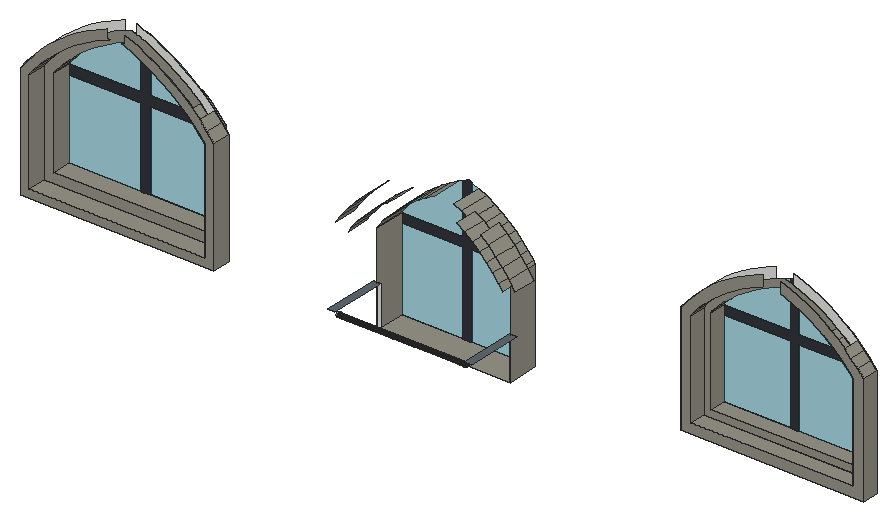
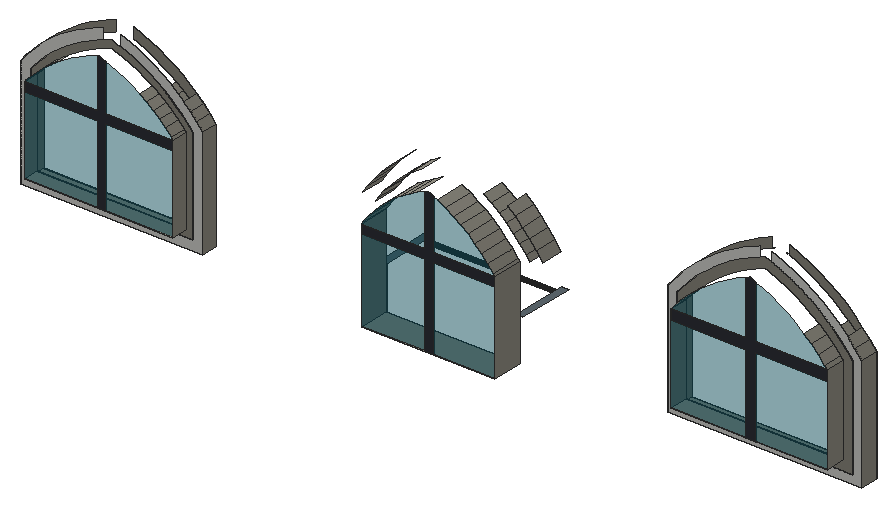
# SketchUp Ruby script. Lengths in inches.
U = 1.inch
M = Sketchup.active_model
def pt(a) = Geom::Point3d.new(a.map { |v| v * U })
def face(e, loops, mat)
  f = e.add_face(loops[0].map { |a| pt(a) })
  loops[1..].each { |l| e.add_face(l.map { |a| pt(a) }).erase! }
  f.material = f.back_material = mat if mat
  f
end
# faces: each face lists its corners as indices into pts; further lists are holes
def faces(e, pts, list, mat = nil) = list.each { |f| face(e, (f[0].is_a?(Array) ? f : [f]).map { |l| l.map { |i| pts[i] } }, mat) }
# xy, xz, yz: faces in a plane at the given z, y or x. An outline is a flat list of corners, or four numbers for a rectangle; further outlines are holes
def ring(l) = l.size == 4 ? [[l[0], l[1]], [l[2], l[1]], [l[2], l[3]], [l[0], l[3]]] : l.each_slice(2).to_a
def flat(e, list, mat, &to3) = list.each { |f| face(e, (f[0].is_a?(Array) ? f : [f]).map { |l| ring(l).map { |u, v| to3.(u, v) } }, mat) }
def xy(e, z, list, mat = nil) = flat(e, list, mat) { |x, y| [x, y, z] }
def xz(e, y, list, mat = nil) = flat(e, list, mat) { |x, z| [x, y, z] }
def yz(e, x, list, mat = nil) = flat(e, list, mat) { |y, z| [x, y, z] }
def lines(e, pts, list) = list.each { |a, b| e.add_line(pt(pts[a]), pt(pts[b])) }
# prism: a flat outline (further loops are holes) pulled along v
def prism(e, loops, v, mat = nil)
  f = face(e, loops, mat); d = Geom::Vector3d.new(v.map { |x| x * U })
  f.pushpull(f.normal.samedirection?(d) ? d.length : -d.length)
end
def box(e, o, s, mat = nil) = prism(e, [[o, [o[0] + s[0], o[1], o[2]], [o[0] + s[0], o[1] + s[1], o[2]], [o[0], o[1] + s[1], o[2]]]], [0, 0, s[2]], mat)
def at(x, y, z, deg = 0) = Geom::Transformation.translation(pt([x, y, z])) * Geom::Transformation.rotation(ORIGIN, Z_AXIS, deg.degrees)
def axes(o, x, y, z) = Geom::Transformation.new([*x, 0, *y, 0, *z, 0, *pt(o).to_a, 1])
def part(name) = M.definitions.add(name)
# library, detail: a bought-in or finely detailed component or shape, given as its bounding box
def library(name, o, s) = part(name).tap { |d| box(d.entities, o, s) }
def detail(e, o, s) = box(e.add_group.entities, o, s)
def put(e, d, t, mat = nil) = e.add_instance(d, t).tap { |i| i.material = mat if mat }
def group(e, t, mat = nil) = e.add_group.tap { |g| g.transformation = t; g.material = mat if mat }.entities
root = M.entities
M.materials.add("[Color M07]").color = [58, 58, 58]
M.materials.add("[Formica Graystone]").color = [149, 146, 135]
M.materials.add("[Formica Laminate Dark]").color = [50, 53, 60]
M.materials.add("[Formica Speckled Grey]").color = [94, 105, 111]
M.materials.add("[Translucent Glass Tinted]").color = [4, 106, 127]
M.materials["[Translucent Glass Tinted]"].alpha = 0.48
xy(root,560.54,[[225.01,144.04,289.71,158.91]],"[Formica Graystone]")
xy(root,564.14,[[366.85,150.49,455.33,158.3]],"[Formica Graystone]")
xy(root,564.93,[[59.5,135.04,153.15,144.04]],"[Formica Graystone]")
xy(root,569.11,[[371.82,150.49,450.36,158.3]],"[Formica Graystone]")
xy(root,569.18,[[63.76,135.04,148.9,144.04]],"[Formica Graystone]")
xy(root,572.37,[[375.08,158.3,447.11,166.11]],"[Formica Graystone]")
xy(root,573.78,[[68.36,144.04,144.3,153.35]],"[Formica Graystone]")
xy(root,578.67,[[230.48,117.55,230.64,117.57,230.79,117.63,230.92,117.73,231.02,117.86,231.08,118.01,231.1,118.17,231.08,118.33,231.02,118.48,230.92,118.61,230.79,118.71,230.64,118.77,230.48,118.8,230.3125,118.77,230.16,118.71,230.03,118.61,229.93,118.48,229.87,118.33,229.85,118.17,229.87,118.01,229.93,117.86,230.03,117.73,230.16,117.63,230.3125,117.57]])
xy(root,578.86,[[228.1,117.55,228.26,117.57,228.41,117.63,228.54,117.73,228.64,117.86,228.7,118.01,228.73,118.17,228.7,118.33,228.64,118.48,228.54,118.61,228.41,118.71,228.26,118.77,228.1,118.8,227.9375,118.77,227.79,118.71,227.66,118.61,227.56,118.48,227.5,118.33,227.48,118.17,227.5,118.01,227.56,117.86,227.66,117.73,227.79,117.63,227.9375,117.57],[261.35,117.55,261.51,117.57,261.66,117.63,261.79,117.73,261.89,117.86,261.95,118.01,261.98,118.17,261.95,118.33,261.89,118.48,261.79,118.61,261.66,118.71,261.51,118.77,261.35,118.8,261.1875,118.77,261.04,118.71,260.91,118.61,260.81,118.48,260.75,118.33,260.73,118.17,260.75,118.01,260.81,117.86,260.91,117.73,261.04,117.63,261.1875,117.57],[283.35,117.55,283.51,117.57,283.66,117.63,283.79,117.73,283.89,117.86,283.95,118.01,283.98,118.17,283.95,118.33,283.89,118.48,283.79,118.61,283.66,118.71,283.51,118.77,283.35,118.8,283.1875,118.77,283.04,118.71,282.91,118.61,282.81,118.48,282.75,118.33,282.73,118.17,282.75,118.01,282.81,117.86,282.91,117.73,283.04,117.63,283.1875,117.57]])
xy(root,578.98,[[235.23,117.55,235.39,117.57,235.54,117.63,235.67,117.73,235.77,117.86,235.83,118.01,235.85,118.17,235.83,118.33,235.77,118.48,235.67,118.61,235.54,118.71,235.39,118.77,235.23,118.8,235.0625,118.77,234.91,118.71,234.78,118.61,234.68,118.48,234.62,118.33,234.6,118.17,234.62,118.01,234.68,117.86,234.78,117.73,234.91,117.63,235.0625,117.57]])
xy(root,579.09,[[242.35,117.55,242.51,117.57,242.66,117.63,242.79,117.73,242.89,117.86,242.95,118.01,242.98,118.17,242.95,118.33,242.89,118.48,242.79,118.61,242.66,118.71,242.51,118.77,242.35,118.8,242.1875,118.77,242.04,118.71,241.91,118.61,241.81,118.48,241.75,118.33,241.73,118.17,241.75,118.01,241.81,117.86,241.91,117.73,242.04,117.63,242.1875,117.57]])
xy(root,579.11,[[263.73,117.55,263.89,117.57,264.04,117.63,264.17,117.73,264.27,117.86,264.33,118.01,264.35,118.17,264.33,118.33,264.27,118.48,264.17,118.61,264.04,118.71,263.89,118.77,263.73,118.8,263.5625,118.77,263.41,118.71,263.28,118.61,263.18,118.48,263.12,118.33,263.1,118.17,263.12,118.01,263.18,117.86,263.28,117.73,263.41,117.63,263.5625,117.57]])
xy(root,579.17,[[256.6,117.55,256.76,117.57,256.91,117.63,257.04,117.73,257.14,117.86,257.2,118.01,257.23,118.17,257.2,118.33,257.14,118.48,257.04,118.61,256.91,118.71,256.76,118.77,256.6,118.8,256.4375,118.77,256.29,118.71,256.16,118.61,256.06,118.48,256,118.33,255.98,118.17,256,118.01,256.06,117.86,256.16,117.73,256.29,117.63,256.4375,117.57],[258.98,117.55,259.14,117.57,259.29,117.63,259.42,117.73,259.52,117.86,259.58,118.01,259.6,118.17,259.58,118.33,259.52,118.48,259.42,118.61,259.29,118.71,259.14,118.77,258.98,118.8,258.8125,118.77,258.66,118.71,258.53,118.61,258.43,118.48,258.37,118.33,258.35,118.17,258.37,118.01,258.43,117.86,258.53,117.73,258.66,117.63,258.8125,117.57]])
xy(root,579.29,[[288.29,117.55,288.45,117.57,288.6,117.63,288.73,117.73,288.83,117.86,288.89,118.01,288.91,118.17,288.89,118.33,288.83,118.48,288.73,118.61,288.6,118.71,288.45,118.77,288.29,118.8,288.125,118.77,287.98,118.71,287.85,118.61,287.75,118.48,287.68,118.33,287.66,118.17,287.68,118.01,287.75,117.86,287.85,117.73,287.98,117.63,288.125,117.57]])
xy(root,579.32,[[237.6,117.55,237.76,117.57,237.91,117.63,238.04,117.73,238.14,117.86,238.2,118.01,238.23,118.17,238.2,118.33,238.14,118.48,238.04,118.61,237.91,118.71,237.76,118.77,237.6,118.8,237.4375,118.77,237.29,118.71,237.16,118.61,237.06,118.48,237,118.33,236.98,118.17,237,118.01,237.06,117.86,237.16,117.73,237.29,117.63,237.4375,117.57],[244.73,117.55,244.89,117.57,245.04,117.63,245.17,117.73,245.27,117.86,245.33,118.01,245.35,118.17,245.33,118.33,245.27,118.48,245.17,118.61,245.04,118.71,244.89,118.77,244.73,118.8,244.5625,118.77,244.41,118.71,244.28,118.61,244.18,118.48,244.12,118.33,244.1,118.17,244.12,118.01,244.18,117.86,244.28,117.73,244.41,117.63,244.5625,117.57],[247.1,117.55,247.26,117.57,247.41,117.63,247.54,117.73,247.64,117.86,247.7,118.01,247.73,118.17,247.7,118.33,247.64,118.48,247.54,118.61,247.41,118.71,247.26,118.77,247.1,118.8,246.9375,118.77,246.79,118.71,246.66,118.61,246.56,118.48,246.5,118.33,246.48,118.17,246.5,118.01,246.56,117.86,246.66,117.73,246.79,117.63,246.9375,117.57],[285.98,117.55,286.14,117.57,286.29,117.63,286.42,117.73,286.52,117.86,286.58,118.01,286.6,118.17,286.58,118.33,286.52,118.48,286.42,118.61,286.29,118.71,286.14,118.77,285.98,118.8,285.8125,118.77,285.66,118.71,285.53,118.61,285.43,118.48,285.37,118.33,285.35,118.17,285.37,118.01,285.43,117.86,285.53,117.73,285.66,117.63,285.8125,117.57]])
xy(root,579.54,[[232.85,117.55,233.01,117.57,233.16,117.63,233.29,117.73,233.39,117.86,233.45,118.01,233.48,118.17,233.45,118.33,233.39,118.48,233.29,118.61,233.16,118.71,233.01,118.77,232.85,118.8,232.6875,118.77,232.54,118.71,232.41,118.61,232.31,118.48,232.25,118.33,232.23,118.17,232.25,118.01,232.31,117.86,232.41,117.73,232.54,117.63,232.6875,117.57],[239.98,117.55,240.14,117.57,240.29,117.63,240.42,117.73,240.52,117.86,240.58,118.01,240.6,118.17,240.58,118.33,240.52,118.48,240.42,118.61,240.29,118.71,240.14,118.77,239.98,118.8,239.8125,118.77,239.66,118.71,239.53,118.61,239.43,118.48,239.37,118.33,239.35,118.17,239.37,118.01,239.43,117.86,239.53,117.73,239.66,117.63,239.8125,117.57],[249.48,117.55,249.64,117.57,249.79,117.63,249.92,117.73,250.02,117.86,250.08,118.01,250.1,118.17,250.08,118.33,250.02,118.48,249.92,118.61,249.79,118.71,249.64,118.77,249.48,118.8,249.3125,118.77,249.16,118.71,249.03,118.61,248.93,118.48,248.87,118.33,248.85,118.17,248.87,118.01,248.93,117.86,249.03,117.73,249.16,117.63,249.3125,117.57],[251.85,117.55,252.01,117.57,252.16,117.63,252.29,117.73,252.39,117.86,252.45,118.01,252.48,118.17,252.45,118.33,252.39,118.48,252.29,118.61,252.16,118.71,252.01,118.77,251.85,118.8,251.6875,118.77,251.54,118.71,251.41,118.61,251.31,118.48,251.25,118.33,251.23,118.17,251.25,118.01,251.31,117.86,251.41,117.73,251.54,117.63,251.6875,117.57],[254.23,117.55,254.39,117.57,254.54,117.63,254.67,117.73,254.77,117.86,254.83,118.01,254.85,118.17,254.83,118.33,254.77,118.48,254.67,118.61,254.54,118.71,254.39,118.77,254.23,118.8,254.0625,118.77,253.91,118.71,253.78,118.61,253.68,118.48,253.62,118.33,253.6,118.17,253.62,118.01,253.68,117.86,253.78,117.73,253.91,117.63,254.0625,117.57],
  [266.1,117.55,266.26,117.57,266.41,117.63,266.54,117.73,266.64,117.86,266.7,118.01,266.73,118.17,266.7,118.33,266.64,118.48,266.54,118.61,266.41,118.71,266.26,118.77,266.1,118.8,265.9375,118.77,265.79,118.71,265.66,118.61,265.56,118.48,265.5,118.33,265.48,118.17,265.5,118.01,265.56,117.86,265.66,117.73,265.79,117.63,265.9375,117.57],[268.48,117.55,268.64,117.57,268.79,117.63,268.92,117.73,269.02,117.86,269.08,118.01,269.1,118.17,269.08,118.33,269.02,118.48,268.92,118.61,268.79,118.71,268.64,118.77,268.48,118.8,268.3125,118.77,268.16,118.71,268.03,118.61,267.93,118.48,267.87,118.33,267.85,118.17,267.87,118.01,267.93,117.86,268.03,117.73,268.16,117.63,268.3125,117.57],[270.85,117.55,271.01,117.57,271.16,117.63,271.29,117.73,271.39,117.86,271.45,118.01,271.48,118.17,271.45,118.33,271.39,118.48,271.29,118.61,271.16,118.71,271.01,118.77,270.85,118.8,270.6875,118.77,270.54,118.71,270.41,118.61,270.31,118.48,270.25,118.33,270.23,118.17,270.25,118.01,270.31,117.86,270.41,117.73,270.54,117.63,270.6875,117.57],[275.6,117.55,275.76,117.57,275.91,117.63,276.04,117.73,276.14,117.86,276.2,118.01,276.23,118.17,276.2,118.33,276.14,118.48,276.04,118.61,275.91,118.71,275.76,118.77,275.6,118.8,275.4375,118.77,275.29,118.71,275.16,118.61,275.06,118.48,275,118.33,274.98,118.17,275,118.01,275.06,117.86,275.16,117.73,275.29,117.63,275.4375,117.57],[278.04,117.55,278.2,117.57,278.35,117.63,278.48,117.73,278.58,117.86,278.64,118.01,278.66,118.17,278.64,118.33,278.58,118.48,278.48,118.61,278.35,118.71,278.2,118.77,278.04,118.8,277.875,118.77,277.73,118.71,277.6,118.61,277.5,118.48,277.43,118.33,277.41,118.17,277.43,118.01,277.5,117.86,277.6,117.73,277.73,117.63,277.875,117.57]])
xy(root,579.76,[[273.23,117.55,273.39,117.57,273.54,117.63,273.67,117.73,273.77,117.86,273.83,118.01,273.85,118.17,273.83,118.33,273.77,118.48,273.67,118.61,273.54,118.71,273.39,118.77,273.23,118.8,273.0625,118.77,272.91,118.71,272.78,118.61,272.68,118.48,272.62,118.33,272.6,118.17,272.62,118.01,272.68,117.86,272.78,117.73,272.91,117.63,273.0625,117.57],[280.54,117.55,280.7,117.57,280.85,117.63,280.98,117.73,281.08,117.86,281.14,118.01,281.16,118.17,281.14,118.33,281.08,118.48,280.98,118.61,280.85,118.71,280.7,118.77,280.54,118.8,280.375,118.77,280.23,118.71,280.1,118.61,280,118.48,279.93,118.33,279.91,118.17,279.93,118.01,280,117.86,280.1,117.73,280.23,117.63,280.375,117.57]])
xy(root,581.29,[[223.35,116.47,226.66,144.04],[289.43,116.47,292.74,144.04]],"[Formica Speckled Grey]")
xz(root,135.04,[[59.5,564.93,153.15,564.93,153.15,619.89,149.79,623.99,146.23,627.91,142.46,631.63,138.5,635.15,134.35,638.45,130.04,641.52,125.57,644.37,120.95,646.97,116.21,649.32,111.34,651.41,110.11,651.87,110.11,647.8,108.86,647.8,109.76,647.46,114.42,645.46,118.97,643.21,123.38,640.72,127.66,638,131.79,635.05,135.76,631.89,139.55,628.53,143.16,624.96,146.57,621.21,148.9,618.375,148.9,569.18,63.76,569.18,63.76,618.51,66.06,621.43,69.41,625.23,72.98,628.83,76.75,632.21,80.71,635.38,84.84,638.3125,89.13,641,93.58,643.45,98.15,645.63,102.84,647.54,101.22,647.54,101.22,651.47,96.43,649.52,91.63,647.23,86.98,644.67,82.48,641.85,78.15,638.78,74,635.46,70.05,631.91,66.31,628.13,62.79,624.15,59.5,619.98]],"[Formica Graystone]")
xz(root,144.04,[[225.01,560.54,226.66,581.29],[289.43,560.54,289.71,581.29],[59.5,564.93,59.5,619.98,62.79,624.15,66.31,628.13,70.05,631.91,74,635.46,78.15,638.78,82.48,641.85,86.98,644.67,91.63,647.23,96.43,649.52,101.35,651.53,102.84,652.04,102.84,647.54,98.15,645.63,93.58,643.45,89.13,641,84.84,638.3125,80.71,635.38,76.75,632.21,72.98,628.83,69.41,625.23,66.06,621.43,63.76,618.51,63.76,569.18,148.9,569.18,148.9,618.375,146.57,621.21,143.16,624.96,139.55,628.53,135.76,631.89,131.79,635.05,127.66,638,123.38,640.72,118.97,643.21,114.42,645.46,109.76,647.46,108.86,647.8,108.86,652.33,111.34,651.41,116.21,649.32,120.95,646.97,125.57,644.37,130.04,641.52,134.35,638.45,138.5,635.15,142.46,631.63,146.23,627.91,149.79,623.99,153.15,619.89,153.15,564.93]])
xz(root,144.04,[[[63.76,569.18,148.9,569.18,148.9,618.375,146.57,621.21,143.16,624.96,139.55,628.53,135.76,631.89,131.79,635.05,127.66,638,123.38,640.72,118.97,643.21,114.42,645.46,109.76,647.46,108.86,647.8,106.32,648.74,102.84,647.54,98.15,645.63,93.58,643.45,89.13,641,84.84,638.3125,80.71,635.38,76.75,632.21,72.98,628.83,69.41,625.23,66.06,621.43,63.76,618.51],[68.36,573.78,68.36,616.91,69.59,618.48,72.77,622.08,76.15,625.49,79.73,628.7,83.48,631.7,87.39,634.49,91.46,637.04,95.67,639.35,100.01,641.42,104.46,643.23,106.26,643.85,108.06,643.19,112.49,641.28,116.8125,639.14,121.02,636.77,125.09,634.18,129.02,631.38,132.8,628.37,136.41,625.17,139.84,621.78,143.09,618.21,144.3,616.73,144.3,573.78]]],"[Formica Graystone]")
xz(root,150.49,[[366.85,564.14,455.33,564.14,455.33,617.39,452.47,620.88,449.43,624.21,446.21,627.37,442.83,630.36,439.29,633.15,435.61,635.76,431.8,638.16,427.86,640.36,423.8,642.34,419.65,644.1,415.41,645.63,415.41,640.35,417.84,639.47,421.74,637.81,425.55,635.95,429.26,633.89,432.85,631.625,436.32,629.17,439.64,626.54,442.83,623.73,445.85,620.76,448.72,617.63,450.36,615.62,450.36,569.11,371.82,569.11,371.82,615.6,373.47,617.6,376.35,620.72,379.39,623.6875,382.58,626.49,385.91,629.12,389.375,631.57,392.97,633.83,396.67,635.9,400.48,637.77,404.39,639.44,406.79,640.32,406.79,645.61,402.55,644.0625,398.41,642.29,394.36,640.3,390.43,638.1,386.61,635.7,382.93,633.1,379.39,630.31,376.01,627.33,372.78,624.18,369.73,620.87,366.85,617.39]],"[Formica Graystone]")
xz(root,153.35,[[103.16,573.78,107.82,573.78,107.82,612,144.3,612,144.3,616.73,144.15,616.91,107.82,616.91,107.82,643.28,106.26,643.85,104.46,643.23,103.16,642.71,103.16,616.91,68.36,616.91,68.36,612,103.16,612]],"[Formica Laminate Dark]")
xz(root,153.35,[[68.36,573.78,103.16,612],[107.82,573.78,144.3,612],[68.36,616.91,103.16,616.91,103.16,642.71,100.01,641.42,95.67,639.35,91.46,637.04,87.39,634.49,83.48,631.7,79.73,628.7,76.15,625.49,72.77,622.08,69.59,618.48],[107.82,616.91,144.15,616.91,143.09,618.21,139.84,621.78,136.41,625.17,132.8,628.37,129.02,631.38,125.09,634.18,121.02,636.77,116.8125,639.14,112.49,641.28,108.06,643.19,107.82,643.28]],"[Translucent Glass Tinted]")
xz(root,158.3,[[366.85,564.14,366.85,617.39,369.73,620.87,372.78,624.18,376.01,627.33,379.39,630.31,382.93,633.1,386.61,635.7,390.43,638.1,394.36,640.3,398.41,642.29,402.55,644.0625,406.79,645.61,406.79,640.32,404.39,639.44,400.48,637.77,396.67,635.9,392.97,633.83,389.375,631.57,385.91,629.12,382.58,626.49,379.39,623.6875,376.35,620.72,373.47,617.6,371.82,615.6,371.82,569.11,450.36,569.11,450.36,615.62,448.72,617.63,445.85,620.76,442.83,623.73,439.64,626.54,436.32,629.17,432.85,631.625,429.26,633.89,425.55,635.95,421.74,637.81,417.84,639.47,415.41,640.35,415.41,645.63,419.65,644.1,423.8,642.34,427.86,640.36,431.8,638.16,435.61,635.76,439.29,633.15,442.83,630.36,446.21,627.37,449.43,624.21,452.47,620.88,455.33,617.39,455.33,564.14]])
xz(root,158.3,[[[371.82,569.11,450.36,569.11,450.36,615.62,448.72,617.63,445.85,620.76,442.83,623.73,439.64,626.54,436.32,629.17,432.85,631.625,429.26,633.89,425.55,635.95,421.74,637.81,417.84,639.47,415.41,640.35,413.85,640.92,411.11,641.74,408.37,640.9,406.79,640.32,404.39,639.44,400.48,637.77,396.67,635.9,392.97,633.83,389.375,631.57,385.91,629.12,382.58,626.49,379.39,623.6875,376.35,620.72,373.47,617.6,371.82,615.6],[375.08,572.37,375.08,614.43,375.92,615.46,378.68,618.45,381.6,621.3,384.66,623.99,387.86,626.51,391.18,628.86,394.63,631.03,398.18,633.02,401.84,634.82,405.59,636.42,409.41,637.82,411.11,638.34,412.82,637.83,416.65,636.44,420.39,634.85,424.05,633.07,427.6,631.09,431.04,628.92,434.37,626.57,437.56,624.04,440.61,621.35,443.51,618.5,446.26,615.5,447.11,614.45,447.11,572.37]]],"[Formica Graystone]")
xz(root,158.91,[[254.77,560.54,259.04,560.54,259.04,600.52,289.71,600.52,289.71,604.82,259.04,604.82,259.04,629.79,258.17,630.16,257.48,630.4,256.79,630.13,254.77,629.22,254.77,604.82,225.01,604.82,225.01,600.52,254.77,600.52]],"[Formica Laminate Dark]")
xz(root,158.91,[[225.01,560.54,254.77,600.52],[259.04,560.54,289.71,600.52],[225.01,604.82,254.77,604.82,254.77,629.22,252.76,628.31,248.84,626.24,245.05,623.95,241.4,621.4375,237.91,618.71,234.59,615.78,231.45,612.66,228.5,609.35,225.75,605.875],[259.04,604.82,289.71,604.82,289.71,605.08,288.92,606.28,286.27,609.77,283.39,613.09,280.31,616.21,277.03,619.12,273.56,621.8125,269.93,624.27,266.14,626.49,262.22,628.45,259.04,629.79]],"[Translucent Glass Tinted]")
xz(root,166.11,[[407.5,572.37,411.64,572.37,411.64,610.09,447.11,610.09,447.11,614.45,446.89,614.43,411.64,614.43,411.64,638.18,411.11,638.34,409.41,637.82,407.5,637.12,407.5,614.43,375.08,614.43,375.08,610.09,407.5,610.09]],"[Formica Laminate Dark]")
xz(root,166.11,[[375.08,572.37,407.5,610.09],[411.64,572.37,447.11,610.09],[375.08,614.43,407.5,614.43,407.5,637.12,405.59,636.42,401.84,634.82,398.18,633.02,394.63,631.03,391.18,628.86,387.86,626.51,384.66,623.99,381.6,621.3,378.68,618.45,375.92,615.46],[411.64,614.43,446.89,614.43,447.11,614.45,446.26,615.5,443.51,618.5,440.61,621.35,437.56,624.04,434.37,626.57,431.04,628.92,427.6,631.09,424.05,633.07,420.39,634.85,416.65,636.44,412.82,637.83,411.64,638.18]],"[Translucent Glass Tinted]")
yz(root,59.5,[[135.04,564.93,144.04,619.98]],"[Formica Graystone]")
yz(root,63.76,[[135.04,569.18,144.04,618.51]],"[Formica Graystone]")
yz(root,68.36,[[144.04,573.78,153.35,616.91]],"[Formica Graystone]")
yz(root,144.3,[[144.04,573.78,153.35,616.73]],"[Formica Graystone]")
yz(root,148.9,[[135.04,569.18,144.04,618.375]],"[Formica Graystone]")
yz(root,153.15,[[135.04,564.93,144.04,619.89]],"[Formica Graystone]")
yz(root,225.01,[[144.04,560.54,158.91,604.82]],"[Formica Graystone]")
yz(root,226.66,[[118.19,578.44,117.96,578.47,117.75,578.56,117.57,578.7,117.43,578.88,117.34,579.09,117.31,579.32,117.34,579.54,117.43,579.76,117.57,579.9375,117.75,580.08,117.96,580.16,118.19,580.19,118.41,580.16,118.62,580.08,118.8,579.9375,118.94,579.76,119.03,579.54,119.06,579.32,119.03,579.09,118.94,578.88,118.8,578.7,118.62,578.56,118.41,578.47]])
yz(root,289.71,[[144.04,560.54,158.91,605.08]],"[Formica Graystone]")
yz(root,366.85,[[150.49,564.14,158.3,617.39]],"[Formica Graystone]")
yz(root,371.82,[[150.49,569.11,158.3,615.6]],"[Formica Graystone]")
yz(root,375.08,[[158.3,572.37,166.11,614.43]],"[Formica Graystone]")
yz(root,447.11,[[158.3,572.37,166.11,614.45]],"[Formica Graystone]")
yz(root,450.36,[[150.49,569.11,158.3,615.62]],"[Formica Graystone]")
yz(root,455.33,[[150.49,564.14,158.3,617.39]],"[Formica Graystone]")
p = [[226.66,117.96,578.47],[226.66,118.19,578.44],[289.43,118.19,578.44],[289.43,117.96,578.47],[226.66,118.41,578.47],[289.43,118.41,578.47],
  [226.66,117.75,578.56],[289.43,117.75,578.56],[226.66,118.62,578.56],[289.43,118.62,578.56],[226.66,117.57,578.7],[289.43,117.57,578.7],
  [288.45,117.57,578.7],[288.125,117.57,578.7],[286.14,117.57,578.7],[285.8125,117.57,578.7],[283.51,117.57,578.7],[283.1875,117.57,578.7],
  [280.7,117.57,578.7],[280.375,117.57,578.7],[278.2,117.57,578.7],[277.875,117.57,578.7],[275.76,117.57,578.7],[275.4375,117.57,578.7],
  [273.39,117.57,578.7],[273.0625,117.57,578.7],[271.01,117.57,578.7],[270.6875,117.57,578.7],[268.64,117.57,578.7],[268.3125,117.57,578.7],
  [266.26,117.57,578.7],[265.9375,117.57,578.7],[263.89,117.57,578.7],[263.5625,117.57,578.7],[261.51,117.57,578.7],[261.1875,117.57,578.7],
  [259.14,117.57,578.7],[258.8125,117.57,578.7],[256.76,117.57,578.7],[256.4375,117.57,578.7],[254.39,117.57,578.7],[254.0625,117.57,578.7],
  [252.01,117.57,578.7],[251.6875,117.57,578.7],[249.64,117.57,578.7],[249.3125,117.57,578.7],[247.26,117.57,578.7],[246.9375,117.57,578.7],
  [244.89,117.57,578.7],[244.5625,117.57,578.7],[242.51,117.57,578.7],[242.1875,117.57,578.7],[240.14,117.57,578.7],[239.8125,117.57,578.7],
  [237.76,117.57,578.7],[237.4375,117.57,578.7],[235.39,117.57,578.7],[235.0625,117.57,578.7],[233.01,117.57,578.7],[232.6875,117.57,578.7],
  [228.26,117.57,578.7],[227.9375,117.57,578.7],[226.66,118.8,578.7],[289.43,118.8,578.7],[226.66,117.43,578.88],[289.43,117.43,578.88],
  [226.66,118.94,578.88],[289.43,118.94,578.88],[226.66,117.34,579.09],[289.43,117.34,579.09],[226.66,119.03,579.09],[289.43,119.03,579.09],
  [226.66,117.31,579.32],[289.43,117.31,579.32],[226.66,119.06,579.32],[289.43,119.06,579.32],[226.66,117.34,579.54],[289.43,117.34,579.54],
  [226.66,119.03,579.54],[289.43,119.03,579.54],[226.66,117.43,579.76],[289.43,117.43,579.76],[226.66,118.94,579.76],[289.43,118.94,579.76],
  [226.66,117.57,579.9375],[289.43,117.57,579.9375],[226.66,118.8,579.9375],[289.43,118.8,579.9375],[226.66,117.75,580.08],[289.43,117.75,580.08],
  [226.66,118.62,580.08],[289.43,118.62,580.08],[226.66,117.96,580.16],[289.43,117.96,580.16],[226.66,118.41,580.16],[289.43,118.41,580.16],
  [226.66,118.19,580.19],[289.43,118.19,580.19],[225.75,144.04,605.875],[225.01,144.04,604.82],[225.01,158.91,604.82],[225.75,158.91,605.875],
  [289.71,144.04,605.08],[288.92,144.04,606.28],[288.92,158.91,606.28],[289.71,158.91,605.08],[228.5,144.04,609.35],[228.5,158.91,609.35],
  [286.27,144.04,609.77],[286.27,158.91,609.77],[220.02,144.04,606.39],[221.74,144.04,608.86],[221.74,132.97,608.86],[220.02,132.97,606.39],
  [293,144.04,609.17],[294.7,144.04,606.58],[294.7,132.97,606.58],[293,132.97,609.17],[216.9,144.04,612.46],[213.99,144.04,608.29],
  [213.99,132.97,608.29],[216.9,132.97,612.46],[300.74,144.04,608.39],[297.92,144.04,612.65],[297.92,132.97,612.65],[300.74,132.97,608.39],
  [224.67,144.04,612.57],[224.67,132.97,612.57],[290.15,144.04,612.92],[290.15,132.97,612.92],[231.45,144.04,612.66],[231.45,158.91,612.66],
  [283.39,144.04,613.09],[283.39,158.91,613.09],[220.05,144.04,616.45],[220.05,132.97,616.45],[227.82,144.04,616.09],[227.82,132.97,616.09],
  [294.83,144.04,616.72],[294.83,132.97,616.72],[234.59,144.04,615.78],[234.59,158.91,615.78],[287.06,144.04,616.49],[287.06,132.97,616.49],
  [280.31,144.04,616.21],[280.31,158.91,616.21],[375.92,158.3,615.46],[375.08,158.3,614.43],[375.08,166.11,614.43],[375.92,166.11,615.46],
  [447.11,158.3,614.45],[446.26,158.3,615.5],[446.26,166.11,615.5],[447.11,166.11,614.45],[378.68,158.3,618.45],[378.68,166.11,618.45],
  [443.51,158.3,618.5],[443.51,166.11,618.5],[371.82,158.3,615.6],[373.47,158.3,617.6],[373.47,150.49,617.6],[371.82,150.49,615.6],
  [448.72,158.3,617.63],[450.36,158.3,615.62],[450.36,150.49,615.62],[448.72,150.49,617.63],[237.91,144.04,618.71],[237.91,158.91,618.71],
  [231.17,144.04,619.43],[231.17,132.97,619.43],[277.03,144.04,619.12],[277.03,158.91,619.12],[223.44,144.04,620.24],[223.44,132.97,620.24],
  [283.75,144.04,619.84],[283.75,132.97,619.84],[291.49,144.04,620.58],[291.49,132.97,620.58],[144.3,144.04,616.73],[143.09,144.04,618.21],
  [143.09,153.35,618.21],[144.15,153.35,616.91],[144.3,153.35,616.73],[69.59,144.04,618.48],[68.36,144.04,616.91],[68.36,153.35,616.91],
  [69.59,153.35,618.48],[369.73,158.3,620.87],[366.85,158.3,617.39],[366.85,150.49,617.39],[369.73,150.49,620.87],[455.33,158.3,617.39],
  [452.47,158.3,620.88],[452.47,150.49,620.88],[455.33,150.49,617.39],[376.35,158.3,620.72],[376.35,150.49,620.72],[445.85,158.3,620.76],
  [445.85,150.49,620.76],[139.84,144.04,621.78],[139.84,153.35,621.78],[146.57,144.04,621.21],[148.9,144.04,618.375],[148.9,135.04,618.375],
  [146.57,135.04,621.21],[63.76,144.04,618.51],[66.06,144.04,621.43],[66.06,135.04,621.43],[63.76,135.04,618.51],[72.77,144.04,622.08],
  [72.77,153.35,622.08],[381.6,158.3,621.3],[381.6,166.11,621.3],[440.61,158.3,621.35],[440.61,166.11,621.35],[241.4,144.04,621.4375],
  [241.4,158.91,621.4375],[273.56,144.04,621.8125],[273.56,158.91,621.8125],[234.72,144.04,622.55],[234.72,132.97,622.55],[280.22,144.04,622.97],
  [280.22,132.97,622.97],[153.15,144.04,619.89],[149.79,144.04,623.99],[149.79,135.04,623.99],[153.15,135.04,619.89],[62.79,144.04,624.15],
  [59.5,144.04,619.98],[59.5,135.04,619.98],[62.79,135.04,624.15],[227.05,144.04,623.83],[227.05,132.97,623.83],[287.9,144.04,624.22],
  [287.9,132.97,624.22],[379.39,158.3,623.6875],[379.39,150.49,623.6875],[442.83,158.3,623.73],[442.83,150.49,623.73],[372.78,158.3,624.18],
  [372.78,150.49,624.18],[449.43,158.3,624.21],[449.43,150.49,624.21],[143.16,144.04,624.96],[143.16,135.04,624.96],[384.66,158.3,623.99],
  [384.66,166.11,623.99],[69.41,144.04,625.23],[69.41,135.04,625.23],[245.05,144.04,623.95],[245.05,158.91,623.95],[437.56,158.3,624.04],
  [437.56,166.11,624.04],[136.41,144.04,625.17],[136.41,153.35,625.17],[269.93,144.04,624.27],[269.93,158.91,624.27],[76.15,144.04,625.49],
  [76.15,153.35,625.49],[238.44,144.04,625.46],[238.44,132.97,625.46],[276.5,144.04,625.86],[276.5,132.97,625.86],[382.58,158.3,626.49],
  [382.58,150.49,626.49],[439.64,158.3,626.54],[439.64,150.49,626.54],[230.86,144.04,627.2],[230.86,132.97,627.2],[146.23,144.04,627.91],
  [146.23,135.04,627.91],[248.84,144.04,626.24],[248.84,158.91,626.24],[387.86,158.3,626.51],[387.86,166.11,626.51],[434.37,158.3,626.57],
  [434.37,166.11,626.57],[284.07,144.04,627.61],[284.07,132.97,627.61],[66.31,144.04,628.13],[66.31,135.04,628.13],[376.01,158.3,627.33],
  [376.01,150.49,627.33],[446.21,158.3,627.37],[446.21,150.49,627.37],[266.14,144.04,626.49],[266.14,158.91,626.49],[139.55,144.04,628.53],
  [139.55,135.04,628.53],[72.98,144.04,628.83],[72.98,135.04,628.83],[132.8,144.04,628.37],[132.8,153.35,628.37],[242.33,144.04,628.15],
  [242.33,132.97,628.15],[79.73,144.04,628.7],[79.73,153.35,628.7],[272.59,144.04,628.5],[272.59,132.97,628.5],[252.76,144.04,628.31],
  [252.76,158.91,628.31],[262.22,144.04,628.45],[262.22,158.91,628.45],[385.91,158.3,629.12],[385.91,150.49,629.12],[436.32,158.3,629.17],
  [436.32,150.49,629.17],[391.18,158.3,628.86],[391.18,166.11,628.86],[431.04,158.3,628.92],[431.04,166.11,628.92]]
faces(root,p,[[0,1,2,3],[1,4,5,2],[6,0,3,7],[4,8,9,5],[10,6,7,11,12,13,14,15,16,17,18,19,20,21,22,23,24,25,26,27,28,29,30,31,32,33,34,35,36,37,38,39,40,41,42,43,44,45,46,47,48,49,50,51,52,53,54,55,56,57,58,59,60,61],[8,62,63,9],[64,10,61,60,59,58,57,56,55,54,53,52,51,50,49,48,47,46,45,44,43,42,41,40,39,38,37,36,35,34,33,32,31,30,29,28,27,26,25,24,23,22,21,20,19,18,17,16,15,14,13,12,11,65],[62,66,67,63],
  [68,64,65,69],[66,70,71,67],[72,68,69,73],[70,74,75,71],[76,72,73,77],[74,78,79,75],[80,76,77,81],[78,82,83,79],
  [84,80,81,85],[82,86,87,83],[88,84,85,89],[86,90,91,87],[92,88,89,93],[90,94,95,91],[96,92,93,97],[94,96,97,95]],"[Color M07]")
faces(root,p,[[98,99,100,101],[102,103,104,105],[106,98,101,107],[103,108,109,104],[110,111,112,113],[114,115,116,117],[118,119,120,121],[122,123,124,125],
  [111,126,127,112],[128,114,117,129],[130,106,107,131],[108,132,133,109],[134,118,121,135],[126,136,137,127],[123,138,139,124],[140,130,131,141],
  [142,128,129,143],[132,144,145,133],[146,147,148,149],[150,151,152,153],[154,146,149,155],[151,156,157,152],[158,159,160,161],[162,163,164,165],
  [166,140,141,167],[136,168,169,137],[144,170,171,145],[172,134,135,173],[174,142,143,175],[138,176,177,139],[178,179,180,181,182],[183,184,185,186],
  [187,188,189,190],[191,192,193,194],[159,195,196,160],[197,162,165,198],[179,199,200,180],[201,202,203,204],[205,206,207,208],[209,183,186,210],
  [211,154,155,212],[156,213,214,157],[215,166,167,216],[170,217,218,171],[168,219,220,169],[221,174,175,222],[223,224,225,226],[227,228,229,230],
  [231,172,173,232],[176,233,234,177],[195,235,236,196],[237,197,198,238],[239,187,190,240],[192,241,242,193],[243,201,204,244],[245,211,212,246],
  [206,247,248,207],[249,215,216,250],[213,251,252,214],[199,253,254,200],[217,255,256,218],[257,209,210,258],[219,259,260,220],[261,221,222,262],
  [235,263,264,236],[265,237,238,266],[267,231,232,268],[224,269,270,225],[271,249,250,272],[273,245,246,274],[251,275,276,252],[233,277,278,234],
  [279,227,230,280],[281,239,240,282],[241,283,284,242],[255,285,286,256],[287,243,244,288],[247,289,290,248],[253,291,292,254],[259,293,294,260],
  [295,257,258,296],[297,261,262,298],[299,271,272,300],[285,301,302,286],[263,303,304,264],[305,265,266,306],[307,273,274,308],[275,309,310,276]],"[Formica Graystone]")
